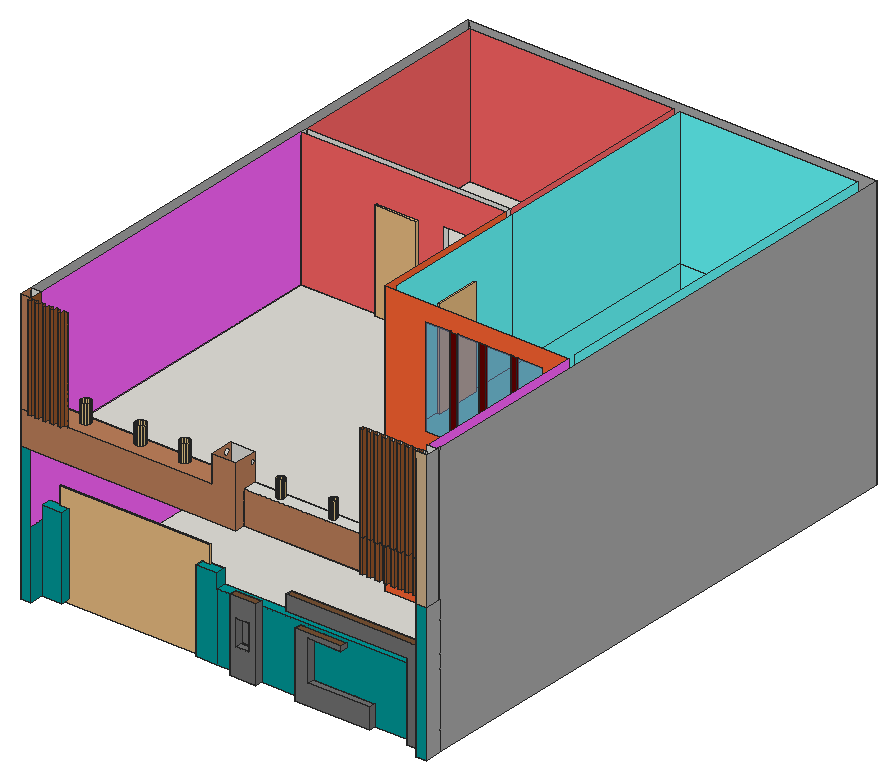
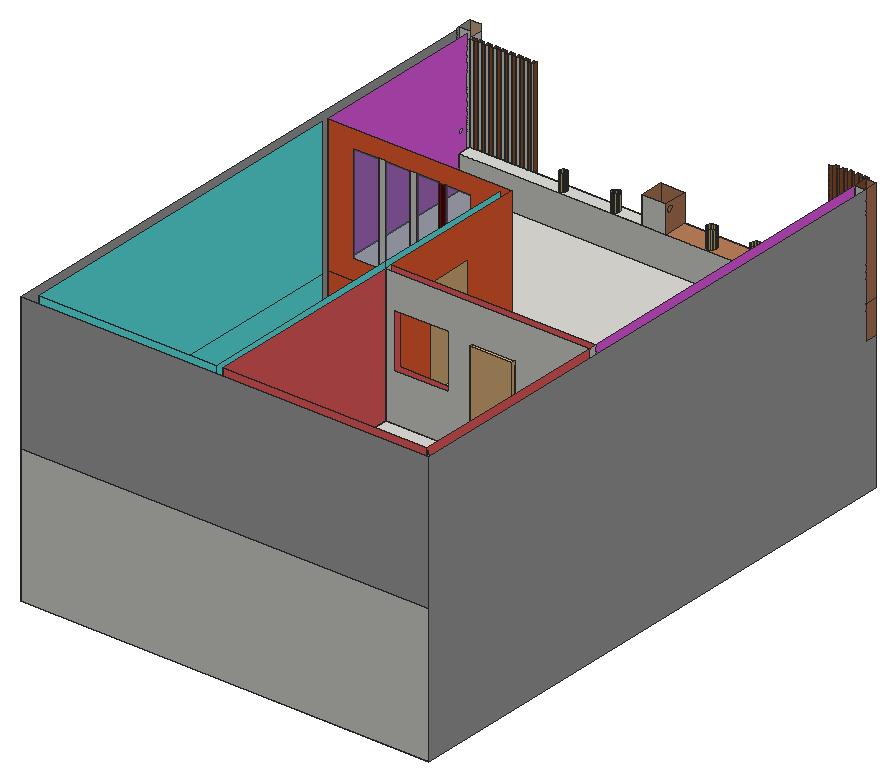
# SketchUp Ruby script. Lengths in inches.
U = 1.inch
M = Sketchup.active_model
def pt(a) = Geom::Point3d.new(a.map { |v| v * U })
def face(e, loops, mat)
  f = e.add_face(loops[0].map { |a| pt(a) })
  loops[1..].each { |l| e.add_face(l.map { |a| pt(a) }).erase! }
  f.material = f.back_material = mat if mat
  f
end
# faces: each face lists its corners as indices into pts; further lists are holes
def faces(e, pts, list, mat = nil) = list.each { |f| face(e, (f[0].is_a?(Array) ? f : [f]).map { |l| l.map { |i| pts[i] } }, mat) }
# xy, xz, yz: faces in a plane at the given z, y or x. An outline is a flat list of corners, or four numbers for a rectangle; further outlines are holes
def ring(l) = l.size == 4 ? [[l[0], l[1]], [l[2], l[1]], [l[2], l[3]], [l[0], l[3]]] : l.each_slice(2).to_a
def flat(e, list, mat, &to3) = list.each { |f| face(e, (f[0].is_a?(Array) ? f : [f]).map { |l| ring(l).map { |u, v| to3.(u, v) } }, mat) }
def xy(e, z, list, mat = nil) = flat(e, list, mat) { |x, y| [x, y, z] }
def xz(e, y, list, mat = nil) = flat(e, list, mat) { |x, z| [x, y, z] }
def yz(e, x, list, mat = nil) = flat(e, list, mat) { |y, z| [x, y, z] }
def lines(e, pts, list) = list.each { |a, b| e.add_line(pt(pts[a]), pt(pts[b])) }
# prism: a flat outline (further loops are holes) pulled along v
def prism(e, loops, v, mat = nil)
  f = face(e, loops, mat); d = Geom::Vector3d.new(v.map { |x| x * U })
  f.pushpull(f.normal.samedirection?(d) ? d.length : -d.length)
end
def box(e, o, s, mat = nil) = prism(e, [[o, [o[0] + s[0], o[1], o[2]], [o[0] + s[0], o[1] + s[1], o[2]], [o[0], o[1] + s[1], o[2]]]], [0, 0, s[2]], mat)
def at(x, y, z, deg = 0) = Geom::Transformation.translation(pt([x, y, z])) * Geom::Transformation.rotation(ORIGIN, Z_AXIS, deg.degrees)
def axes(o, x, y, z) = Geom::Transformation.new([*x, 0, *y, 0, *z, 0, *pt(o).to_a, 1])
def part(name) = M.definitions.add(name)
# library, detail: a bought-in or finely detailed component or shape, given as its bounding box
def library(name, o, s) = part(name).tap { |d| box(d.entities, o, s) }
def detail(e, o, s) = box(e.add_group.entities, o, s)
def put(e, d, t, mat = nil) = e.add_instance(d, t).tap { |i| i.material = mat if mat }
def group(e, t, mat = nil) = e.add_group.tap { |g| g.transformation = t; g.material = mat if mat }.entities
root = M.entities
M.materials.add("[0035_Tan]").color = [210, 180, 140]
M.materials.add("[Color A03]").color = [255, 101, 101]
M.materials.add("[Color A08]1").color = [102, 0, 0]
M.materials.add("[Color B04]").color = [255, 101, 50]
M.materials.add("[Color H03]").color = [101, 255, 255]
M.materials.add("[Color H07]").color = [0, 153, 153]
M.materials.add("[Color K03]").color = [255, 101, 255]
M.materials.add("[Color M03]").color = [170, 170, 170]
M.materials.add("[Color M05]").color = [114, 114, 114]
M.materials.add("[Color M09]").color = [0, 0, 0]
M.materials.add("[Marble Carrara Gold Floor Tile]").color = [225, 223, 217]
M.materials.add("[Sandstone]").color = [118, 81, 52]
M.materials.add("[Stone Brushed Khaki]").color = [226, 197, 133]
M.materials.add("[Translucent Glass Sky Reflection]").color = [126, 138, 183]
M.materials["[Translucent Glass Sky Reflection]"].alpha = 0.52
M.materials.add("[Wood Cherry Original]").color = [152, 86, 42]
M.materials.add("[Wood Veneer 02]").color = [190, 128, 91]
c1 = library("gate",[-28.22,15.88,-5.11],[182.45,4.03,139.23])
c2 = library("DOOR (1)\#1",[0,-8.5,0],[36,11.125,84])
c3 = library("DOOR (1)\#2",[0,-8.5,0],[36,11.125,84])
c4 = library("DOOR (1)",[0,-8.63,0],[36.49,11.68,86.95])
xy(root,0,[[351.25,24,360.25,39],[0.25,27,0.25,519,360.25,519,360.25,39,145.0625,39,145.0625,48,351.25,48,351.25,192.3125,188.875,192.3125,188.875,246.36,194.875,246.36,194.875,198.3125,351.25,198.3125,351.25,510,194.875,510,194.875,282.36,188.875,282.36,188.875,510,9.25,510,9.25,48,27.11,48,27.11,39,9.25,39,9.25,27],[9.25,324.96,75.75,330.96],[111.75,324.96,188.875,330.96]])
xy(root,0,[[9.25,48,351.25,48,351.25,192.3125,188.875,192.3125,188.875,246.36,194.875,246.36,194.875,282.36,188.875,282.36,188.875,324.96,111.75,324.96,111.75,330.96,75.75,330.96,75.75,324.96,9.25,324.96],[194.875,198.3125,351.25,510],[9.25,330.96,188.875,510]],"[Marble Carrara Gold Floor Tile]")
xy(root,0,[[180.02,33,203.03,39],[237.34,33,302.96,39],[335.59,33,351.25,39]],"[Sandstone]")
xy(root,17.83,[[248.65,33,302.96,39]],"[Color M05]")
xy(root,17.875,[[246.73,191.3125,252.73,192.3125],[272.86,191.3125,278.86,192.3125],[300.23,191.3125,306.23,192.3125]])
xy(root,24.41,[[185.3125,33,196.5,39]],"[Color M05]")
xy(root,41.89,[[133.81,324.96,181.81,330.96]])
xy(root,47.22,[[185.3125,33,196.5,39]],"[Color M05]")
xy(root,53.16,[[248.65,33,278.03,39]],"[Color M05]")
xy(root,57.34,[[237.34,33,278.03,39]],"[Sandstone]")
xy(root,60,[[163.53,39,351.25,48]],"[Color H07]")
xy(root,64.125,[[180.02,33,203.03,39]],"[Sandstone]")
xy(root,68.2,[[229.59,33,335.59,39]],"[Color M05]")
xy(root,72,[[9.25,39,27.11,48],[145.0625,39,163.53,48]],"[Color H07]")
xy(root,81.18,[[229.59,33,351.25,39]],"[Sandstone]")
xy(root,84,[[188.875,246.36,194.875,282.36],[75.75,324.96,111.75,330.96]])
xy(root,89.89,[[133.81,324.96,181.81,330.96]])
xy(root,104.8125,[[246.73,191.3125,252.73,192.3125],[272.86,191.3125,278.86,192.3125],[300.23,191.3125,306.23,192.3125]],"[Color A08]1")
xy(root,120,[[351.25,24,360.25,36],[351.25,36,360.25,39],[9.25,39,351.25,48],[188.875,282.36,188.875,330.375,194.875,324.375,194.875,282.36],[9.25,324.96,75.75,330.96],
  [111.75,324.96,188.875,324.96,188.875,330.375,188.29,330.96,111.75,330.96],[188.875,330.375,188.875,330.96,188.29,330.96]])
xy(root,120,[[75.75,324.96,111.75,330.96]],"[Color A03]")
xy(root,120,[[188.875,246.36,194.875,282.36]],"[Color B04]")
xy(root,120,[[9.25,48,351.25,48,351.25,192.3125,188.875,192.3125,188.875,324.96,9.25,324.96],[9.25,330.96,188.875,510]],"[Marble Carrara Gold Floor Tile]")
xy(root,120,[[294.16,33,296.82,36],[300.5,33,304.19,36],[307.88,33,311.57,36],[315.25,33,318.44,36],[321.63,33,324.82,36],
  [328,33,331.19,36],[334.38,33,337.57,36],[340.75,33,343.94,36],[347.13,33,351.25,36]],"[Wood Cherry Original]")
xy(root,120,[[9.25,27,190.02,39],[190.02,36,351.25,39]],"[Wood Veneer 02]")
xy(root,137.875,[[246.73,191.3125,252.73,192.3125],[272.86,191.3125,278.86,192.3125],[300.23,191.3125,306.23,192.3125]])
xy(root,149.4375,[[0.25,27,9.25,39],[294.16,33,296.82,36],[300.5,33,303.66,36],[307.88,33,310.41,36],[315.25,33,317.16,36],
  [321.63,33,323.91,36],[328,33,330.66,36],[334.38,33,337.41,36],[337.41,33,337.57,36],[340.75,33,340.79,36],
  [340.79,33,343.94,36],[343.94,33,344.16,36],[347.13,33,351.25,36],[[190.02,36,351.25,48],[217.02,39.6875,216.19,39.77,215.42,40.0625,214.74,40.55,214.21,41.19,213.87,41.95,213.74,42.77,213.82,43.6,214.11,44.38,214.6,45.05,215.24,45.58,216,45.92,216.82,46.06,217.65,45.98,218.43,45.68,219.1,45.2,219.63,44.55,219.97,43.79,220.11,42.97,220.03,42.14,219.73,41.37,219.25,40.69,218.6,40.16,217.84,39.82],[263.46,39.6875,262.63,39.77,261.85,40.0625,261.18,40.55,260.65,41.19,260.31,41.95,260.17,42.77,260.26,43.6,260.55,44.38,261.04,45.05,261.68,45.58,262.4375,45.92,263.26,46.06,264.09,45.98,264.87,45.68,265.54,45.2,266.07,44.55,266.41,43.79,266.55,42.97,266.46,42.14,266.17,41.37,265.68,40.69,265.04,40.16,264.28,39.82]],[94.51,37.09,93.375,37.24,92.32,37.68,91.41,38.375,90.72,39.28,90.28,40.34,90.13,41.47,90.28,42.6,90.72,43.66,91.41,44.56,92.32,45.26,93.375,45.7,94.51,45.85,95.64,45.7,96.7,45.26,97.6,44.56,98.3,43.66,98.74,42.6,98.89,41.47,98.74,40.34,98.3,39.28,97.6,38.375,96.7,37.68,95.64,37.24],
  [133.45,37.09,132.3125,37.24,131.26,37.68,130.35,38.375,129.66,39.28,129.22,40.34,129.07,41.47,129.22,42.6,129.66,43.66,130.35,44.56,131.26,45.26,132.3125,45.7,133.45,45.85,134.58,45.7,135.64,45.26,136.54,44.56,137.24,43.66,137.67,42.6,137.82,41.47,137.67,40.34,137.24,39.28,136.54,38.375,135.64,37.68,134.58,37.24],[217.02,39.6875,216.19,39.77,215.42,40.0625,214.74,40.55,214.21,41.19,213.87,41.95,213.74,42.77,213.82,43.6,214.11,44.38,214.6,45.05,215.24,45.58,216,45.92,216.82,46.06,217.65,45.98,218.43,45.68,219.1,45.2,219.63,44.55,219.97,43.79,220.11,42.97,220.03,42.14,219.73,41.37,219.25,40.69,218.6,40.16,217.84,39.82],[263.46,39.6875,262.63,39.77,261.85,40.0625,261.18,40.55,260.65,41.19,260.31,41.95,260.17,42.77,260.26,43.6,260.55,44.38,261.04,45.05,261.68,45.58,262.4375,45.92,263.26,46.06,264.09,45.98,264.87,45.68,265.54,45.2,266.07,44.55,266.41,43.79,266.55,42.97,266.46,42.14,266.17,41.37,265.68,40.69,265.04,40.16,264.28,39.82]])
xy(root,149.4375,[[9.25,24,12.5,27],[15.75,24,19,27],[22.25,24,25.5,27],[28.75,24,32,27],[35.25,24,38.5,27],
  [296.82,33,296.91,36],[300.29,33,300.5,36],[303.66,33,304.19,36],[307.04,33,307.88,36],[310.41,33,311.57,36],
  [313.79,33,315.25,36],[317.16,33,318.44,36],[320.54,33,321.63,36],[323.91,33,324.82,36],[327.29,33,328,36],
  [330.66,33,331.19,36],[334.04,33,334.38,36]],"[Wood Cherry Original]")
xy(root,149.4375,[[[9.25,27,169.02,48],[133.45,37.09,132.3125,37.24,131.26,37.68,130.35,38.375,129.66,39.28,129.22,40.34,129.07,41.47,129.22,42.6,129.66,43.66,130.35,44.56,131.26,45.26,132.3125,45.7,133.45,45.85,134.58,45.7,135.64,45.26,136.54,44.56,137.24,43.66,137.67,42.6,137.82,41.47,137.67,40.34,137.24,39.28,136.54,38.375,135.64,37.68,134.58,37.24],[94.51,37.09,93.375,37.24,92.32,37.68,91.41,38.375,90.72,39.28,90.28,40.34,90.13,41.47,90.28,42.6,90.72,43.66,91.41,44.56,92.32,45.26,93.375,45.7,94.51,45.85,95.64,45.7,96.7,45.26,97.6,44.56,98.3,43.66,98.74,42.6,98.89,41.47,98.74,40.34,98.3,39.28,97.6,38.375,96.7,37.68,95.64,37.24],[46.45,37.09,45.3125,37.24,44.26,37.68,43.35,38.375,42.66,39.28,42.22,40.34,42.07,41.47,42.22,42.6,42.66,43.66,43.35,44.56,44.26,45.26,45.3125,45.7,46.45,45.85,47.58,45.7,48.64,45.26,49.54,44.56,50.24,43.66,50.67,42.6,50.82,41.47,50.67,40.34,50.24,39.28,49.54,38.375,48.64,37.68,47.58,37.24]]],"[Wood Veneer 02]")
xz(root,24,[[351.25,120,360.25,240.8125]],"[0035_Tan]")
xz(root,24,[[351.25,0,360.25,120]],"[Color H07]")
xz(root,24,[[9.25,149.4375,12.5,240],[15.75,149.4375,19,240],[22.25,149.4375,25.5,240],[28.75,149.4375,32,240],[35.25,149.4375,38.5,240]],"[Wood Cherry Original]")
xz(root,27,[[9.25,149.4375,12.5,240]])
xz(root,27,[[0.25,0,9.25,120]],"[Color H07]")
xz(root,27,[[12.5,149.4375,15.75,240],[19,149.4375,22.25,240],[25.5,149.4375,28.75,240],[32,149.4375,35.25,240],[38.5,149.4375,41.75,240],
  [41.75,149.4375,42.3125,240]],"[Wood Cherry Original]")
xz(root,27,[[0.25,120,190.02,120,190.02,173.4375,169.02,173.4375,169.02,149.4375,0.25,149.4375],[0.25,149.4375,9.25,240]],"[Wood Veneer 02]")
xz(root,33,[[[180.02,0,203.03,64.125],[185.3125,24.41,196.5,47.22]],[335.59,0,351.25,0,351.25,81.18,229.59,81.18,229.59,68.2,335.59,68.2],[237.34,0,302.96,0,302.96,17.83,248.65,17.83,248.65,53.16,278.03,53.16,278.03,57.34,237.34,57.34]],"[Color M05]")
xz(root,33,[[294.16,120,296.82,149.4375],[300.5,120,304.19,149.4375],[307.88,120,311.57,149.4375],[315.25,120,318.44,149.4375],[321.63,120,324.82,149.4375],
  [328,120,331.19,149.4375],[334.38,120,337.57,149.4375],[340.75,120,343.94,149.4375],[347.13,120,351.25,149.4375],[294.16,149.4375,296.91,234.8125],
  [300.29,149.4375,303.66,234.8125],[307.04,149.4375,310.41,234.8125],[313.79,149.4375,317.16,234.8125],[320.54,149.4375,323.91,234.8125],[327.29,149.4375,330.66,234.8125],
  [334.04,149.4375,337.41,234.8125],[340.79,149.4375,344.16,234.8125],[347.13,149.4375,351.25,234.8125]],"[Wood Cherry Original]")
xz(root,36,[[294.16,120,296.82,149.4375],[300.5,120,304.19,149.4375],[307.88,120,311.57,149.4375],[315.25,120,318.44,149.4375],[321.63,120,324.82,149.4375],
  [328,120,331.19,149.4375],[334.38,120,337.57,149.4375],[340.75,120,343.94,149.4375],[347.13,120,351.25,149.4375],[351.25,120,360.25,240.8125],
  [294.16,149.4375,296.91,234.8125],[300.29,149.4375,303.66,234.8125],[307.04,149.4375,310.41,234.8125],[313.79,149.4375,317.16,234.8125],[320.54,149.4375,323.91,234.8125],
  [327.29,149.4375,330.66,234.8125],[334.04,149.4375,337.41,234.8125],[340.79,149.4375,344.16,234.8125],[347.13,149.4375,351.25,234.8125]])
xz(root,36,[[296.82,120,300.5,149.4375],[304.19,120,307.88,149.4375],[311.57,120,315.25,149.4375],[318.44,120,321.63,149.4375],[324.82,120,328,149.4375],
  [331.19,120,334.38,149.4375],[337.57,120,340.75,149.4375],[343.94,120,347.13,149.4375],[296.91,149.4375,300.29,234.8125],[303.66,149.4375,307.04,234.8125],
  [310.41,149.4375,313.79,234.8125],[317.16,149.4375,320.54,234.8125],[323.91,149.4375,327.29,234.8125],[330.66,149.4375,334.04,234.8125],[337.41,149.4375,340.79,234.8125],
  [344.16,149.4375,347.13,234.8125]],"[Wood Cherry Original]")
xz(root,36,[[190.02,120,294.16,149.4375]],"[Wood Veneer 02]")
xz(root,39,[[[180.02,0,203.03,60],[185.3125,24.41,196.5,47.22]],[237.34,0,237.34,57.34,278.03,57.34,278.03,53.16,248.65,53.16,248.65,17.83,302.96,17.83,302.96,0],[335.59,0,351.25,60],[351.25,0,360.25,120],[180.02,60,203.03,64.125],
  [335.59,60,335.59,68.2,229.59,68.2,229.59,81.18,351.25,81.18,351.25,60],[0.25,149.4375,9.25,240]])
xz(root,39,[[9.25,0,27.11,72],[145.0625,0,163.53,72],[163.53,0,180.02,60],[203.03,0,237.34,0,237.34,57.34,278.03,57.34,278.03,53.16,248.65,53.16,248.65,17.83,302.96,17.83,302.96,0,335.59,0,335.59,60,203.03,60]],"[Color H07]")
xz(root,39,[[185.3125,24.41,196.5,47.22]],"[Color M05]")
xz(root,48,[[9.25,0,27.11,72],[145.0625,0,145.0625,72,163.53,72,163.53,60,351.25,60,351.25,0],[9.25,120,351.25,149.4375],[169.02,149.4375,190.02,173.4375]])
xz(root,191.3125,[[246.73,17.875,252.73,104.8125],[272.86,17.875,278.86,104.8125],[300.23,17.875,306.23,104.8125],[246.73,137.875,252.73,224.8125],[272.86,137.875,278.86,224.8125],
  [300.23,137.875,306.23,224.8125]],"[Color A08]1")
xz(root,192.3125,[[272.86,17.875,278.86,104.8125],[300.23,17.875,306.23,104.8125],[272.86,137.875,278.86,224.8125],[300.23,137.875,306.23,224.8125]])
xz(root,192.3125,[[[188.875,0,351.25,120],[224.8,17.875,328.11,104.8125]],[[188.875,120,351.25,240],[224.8,137.875,328.11,224.8125]]],"[Color B04]")
xz(root,192.3125,[[224.8,17.875,246.73,104.8125],[252.73,17.875,272.86,104.8125],[278.86,17.875,300.23,104.8125],[306.23,17.875,328.11,104.8125],[224.8,137.875,246.73,224.8125],
  [252.73,137.875,272.86,224.8125],[278.86,137.875,300.23,224.8125],[306.23,137.875,328.11,224.8125]],"[Translucent Glass Sky Reflection]")
xz(root,246.36,[[188.875,0,194.875,84],[188.875,120,194.875,204]])
xz(root,282.36,[[188.875,0,194.875,84],[188.875,120,194.875,204]])
xz(root,324.96,[[[9.25,0,75.75,0,75.75,84,111.75,84,111.75,0,188.875,0,188.875,120,9.25,120],[133.81,41.89,181.81,89.89]],[[9.25,120,75.75,120,75.75,204,111.75,204,111.75,120,188.875,120,188.875,240,9.25,240],[133.81,161.89,181.81,209.89]]],"[Color A03]")
xz(root,330.96,[[[9.25,0,9.25,120,188.875,120,188.875,0,111.75,0,111.75,84,75.75,84,75.75,0],[133.81,41.89,181.81,89.89]],[[9.25,120,9.25,240,188.875,240,188.875,120,111.75,120,111.75,204,75.75,204,75.75,120],[133.81,161.89,181.81,209.89]]])
xz(root,510,[[9.25,0,188.875,120],[9.25,120,188.875,240]],"[Color A03]")
xz(root,510,[[194.875,0,351.25,120],[194.875,120,351.25,240]],"[Color H03]")
xz(root,519,[[0.25,0,360.25,120]])
xz(root,519,[[0.25,120,360.25,240]],"[Color M03]")
yz(root,0.25,[[27,0,27,120,39,120,39,240,519,240,519,0]],"[Color M03]")
yz(root,0.25,[[27,120,39,149.4375],[27,149.4375,39,240]],"[Wood Veneer 02]")
yz(root,9.25,[[324.96,0,330.96,120],[324.96,120,330.96,240]])
yz(root,9.25,[[330.96,0,510,120],[330.96,120,510,240]],"[Color A03]")
yz(root,9.25,[[27,0,39,60]],"[Color H07]")
yz(root,9.25,[[48,0,324.96,0,324.96,120,27,120,27,60,39,60,39,72,48,72],[48,120,324.96,120,324.96,240,39,240,39,149.4375,48,149.4375]],"[Color K03]")
yz(root,9.25,[[24,149.4375,27,240],[27,149.4375,39,240]],"[Wood Cherry Original]")
yz(root,12.5,[[24,149.4375,27,240]],"[Wood Cherry Original]")
yz(root,15.75,[[24,149.4375,27,240]],"[Wood Cherry Original]")
yz(root,19,[[24,149.4375,27,240]],"[Wood Cherry Original]")
yz(root,22.25,[[24,149.4375,27,240]],"[Wood Cherry Original]")
yz(root,25.5,[[24,149.4375,27,240]],"[Wood Cherry Original]")
yz(root,27.11,[[39,0,48,72]],"[Color H07]")
yz(root,28.75,[[24,149.4375,27,240]],"[Wood Cherry Original]")
yz(root,32,[[24,149.4375,27,240]],"[Wood Cherry Original]")
yz(root,35.25,[[24,149.4375,27,240]],"[Wood Cherry Original]")
yz(root,38.5,[[24,149.4375,27,240]],"[Wood Cherry Original]")
yz(root,75.75,[[324.96,0,330.96,84],[324.96,120,330.96,204]])
yz(root,111.75,[[324.96,0,330.96,84],[324.96,120,330.96,204]])
yz(root,133.81,[[324.96,41.89,330.96,89.89]])
yz(root,145.0625,[[39,0,48,60],[39,60,48,72]],"[Color H07]")
yz(root,163.53,[[39,60,48,72]],"[Color H07]")
yz(root,169.02,[[[27,149.4375,48,173.4375],[43.19,164.77,43.99,164.88,44.73,165.18,45.36,165.67,45.85,166.3,46.15,167.04,46.26,167.84,46.15,168.63,45.85,169.37,45.36,170,44.73,170.49,43.99,170.79,43.19,170.9,42.4,170.79,41.66,170.49,41.03,170,40.54,169.37,40.24,168.63,40.13,167.84,40.24,167.04,40.54,166.3,41.03,165.67,41.66,165.18,42.4,164.88]]],"[Wood Veneer 02]")
yz(root,180.02,[[33,0,39,64.125]],"[Color M05]")
yz(root,181.81,[[324.96,41.89,330.96,89.89]])
yz(root,185.3125,[[33,24.41,39,47.22]],"[Color M05]")
yz(root,188.875,[[324.96,0,330.96,120],[324.96,120,330.96,240]])
yz(root,188.875,[[330.96,0,510,120],[330.96,120,510,240]],"[Color A03]")
yz(root,188.875,[[192.3125,0,192.3125,120,324.96,120,324.96,0,282.36,0,282.36,84,246.36,84,246.36,0],[192.3125,120,192.3125,240,324.96,240,324.96,120,282.36,120,282.36,204,246.36,204,246.36,120]],"[Color B04]")
yz(root,190.02,[[36,120,39,149.4375]])
yz(root,190.02,[[[27,120,36,120,36,149.4375,48,149.4375,48,173.4375,27,173.4375],[45.4,163.94,44.83,164.02,44.3,164.24,43.85,164.58,43.5,165.04,43.28,165.5625,43.21,166.13,43.28,166.7,43.5,167.22,43.85,167.68,44.3,168.02,44.83,168.24,45.4,168.32,45.96,168.24,46.49,168.02,46.94,167.68,47.29,167.22,47.51,166.7,47.58,166.13,47.51,165.5625,47.29,165.04,46.94,164.58,46.49,164.24,45.96,164.02]]],"[Wood Veneer 02]")
yz(root,194.875,[[198.3125,0,246.36,0,246.36,84,282.36,84,282.36,0,510,0,510,120,198.3125,120],[198.3125,120,246.36,120,246.36,204,282.36,204,282.36,120,324.375,120,324.375,240,198.3125,240],[324.375,120,510,240]],"[Color H03]")
yz(root,196.5,[[33,24.41,39,47.22]],"[Color M05]")
yz(root,203.03,[[33,0,39,64.125]],"[Color M05]")
yz(root,229.59,[[33,68.2,39,81.18]],"[Color M05]")
yz(root,237.34,[[33,0,39,57.34]],"[Color M05]")
yz(root,246.73,[[191.3125,17.875,192.3125,104.8125],[191.3125,137.875,192.3125,224.8125]],"[Color A08]1")
yz(root,248.65,[[33,17.83,39,53.16]],"[Color M05]")
yz(root,252.73,[[191.3125,17.875,192.3125,104.8125],[191.3125,137.875,192.3125,224.8125]],"[Color A08]1")
yz(root,272.86,[[191.3125,17.875,192.3125,104.8125],[191.3125,137.875,192.3125,224.8125]],"[Color A08]1")
yz(root,278.03,[[33,53.16,39,57.34]],"[Color M05]")
yz(root,278.86,[[191.3125,17.875,192.3125,104.8125],[191.3125,137.875,192.3125,224.8125]],"[Color A08]1")
yz(root,294.16,[[33,120,36,149.4375],[33,149.4375,36,234.8125]],"[Wood Cherry Original]")
yz(root,296.82,[[33,120,36,149.4375]],"[Wood Cherry Original]")
yz(root,296.91,[[33,149.4375,36,234.8125]],"[Wood Cherry Original]")
yz(root,300.23,[[191.3125,17.875,192.3125,104.8125],[191.3125,137.875,192.3125,224.8125]],"[Color M09]")
yz(root,300.29,[[33,149.4375,36,234.8125]],"[Wood Cherry Original]")
yz(root,300.5,[[33,120,36,149.4375]],"[Wood Cherry Original]")
yz(root,302.96,[[33,0,39,17.83]],"[Color M05]")
yz(root,303.66,[[33,149.4375,36,234.8125]],"[Wood Cherry Original]")
yz(root,304.19,[[33,120,36,149.4375]],"[Wood Cherry Original]")
yz(root,306.23,[[191.3125,17.875,192.3125,104.8125],[191.3125,137.875,192.3125,224.8125]],"[Color A08]1")
yz(root,307.04,[[33,149.4375,36,234.8125]],"[Wood Cherry Original]")
yz(root,307.88,[[33,120,36,149.4375]],"[Wood Cherry Original]")
yz(root,310.41,[[33,149.4375,36,234.8125]],"[Wood Cherry Original]")
yz(root,311.57,[[33,120,36,149.4375]],"[Wood Cherry Original]")
yz(root,313.79,[[33,149.4375,36,234.8125]],"[Wood Cherry Original]")
yz(root,315.25,[[33,120,36,149.4375]],"[Wood Cherry Original]")
yz(root,317.16,[[33,149.4375,36,234.8125]],"[Wood Cherry Original]")
yz(root,318.44,[[33,120,36,149.4375]],"[Wood Cherry Original]")
yz(root,320.54,[[33,149.4375,36,234.8125]],"[Wood Cherry Original]")
yz(root,321.63,[[33,120,36,149.4375]],"[Wood Cherry Original]")
yz(root,323.91,[[33,149.4375,36,234.8125]],"[Wood Cherry Original]")
yz(root,324.82,[[33,120,36,149.4375]],"[Wood Cherry Original]")
yz(root,327.29,[[33,149.4375,36,234.8125]],"[Wood Cherry Original]")
yz(root,328,[[33,120,36,149.4375]],"[Wood Cherry Original]")
yz(root,330.66,[[33,149.4375,36,234.8125]],"[Wood Cherry Original]")
yz(root,331.19,[[33,120,36,149.4375]],"[Wood Cherry Original]")
yz(root,334.04,[[33,149.4375,36,234.8125]],"[Wood Cherry Original]")
yz(root,334.38,[[33,120,36,149.4375]],"[Wood Cherry Original]")
yz(root,335.59,[[33,0,39,68.2]],"[Color M05]")
yz(root,337.41,[[33,149.4375,36,234.8125]],"[Wood Cherry Original]")
yz(root,337.57,[[33,120,36,149.4375]],"[Wood Cherry Original]")
yz(root,340.75,[[33,120,36,149.4375]],"[Wood Cherry Original]")
yz(root,340.79,[[33,149.4375,36,234.8125]],"[Wood Cherry Original]")
yz(root,343.94,[[33,120,36,149.4375]],"[Wood Cherry Original]")
yz(root,344.16,[[33,149.4375,36,234.8125]],"[Wood Cherry Original]")
yz(root,347.13,[[33,120,36,149.4375],[33,149.4375,36,234.8125]],"[Wood Cherry Original]")
yz(root,351.25,[[33,0,39,81.18],[24,120,33,234.8125],[33,120,36,149.4375],[36,120,48,149.4375],[33,149.4375,36,234.8125],
  [36,149.4375,39,234.8125]])
yz(root,351.25,[[198.3125,0,510,120],[198.3125,120,510,240]],"[Color H03]")
yz(root,351.25,[[24,0,33,60],[24,60,24,120,39,120,39,81.18,33,81.18,33,60]],"[Color H07]")
yz(root,351.25,[[48,0,48,60,39,60,39,120,192.3125,120,192.3125,0],[[48,120,48,149.4375,39,149.4375,39,240,192.3125,240,192.3125,120],[45.4,163.94,45.96,164.02,46.49,164.24,46.94,164.58,47.29,165.04,47.51,165.5625,47.58,166.13,47.51,166.7,47.29,167.22,46.94,167.68,46.49,168.02,45.96,168.24,45.4,168.32,44.83,168.24,44.3,168.02,43.85,167.68,43.5,167.22,43.28,166.7,43.21,166.13,43.28,165.5625,43.5,165.04,43.85,164.58,44.3,164.24,44.83,164.02]]],"[Color K03]")
yz(root,360.25,[[24,0,39,120],[39,0,519,240],[24,120,36,240.8125],[36,120,39,240.9375]],"[Color M03]")
p = [[0.25,519,120],[0.25,519,240],[9.25,510,240],[9.25,510,120],[45.3125,37.24,149.4375],[46.45,37.09,149.4375],
  [46.45,37.09,165.67],[45.3125,37.24,165.67],[47.58,37.24,149.4375],[47.58,37.24,165.67],[93.375,37.24,149.4375],[94.51,37.09,149.4375],
  [94.51,37.09,165.0625],[93.375,37.24,165.0625],[95.64,37.24,149.4375],[95.64,37.24,165.0625],[132.3125,37.24,149.4375],[133.45,37.09,149.4375],
  [133.45,37.09,164.88],[132.3125,37.24,164.88],[134.58,37.24,149.4375],[134.58,37.24,164.88],[44.26,37.68,149.4375],[44.26,37.68,165.67],
  [48.64,37.68,149.4375],[48.64,37.68,165.67],[92.32,37.68,149.4375],[92.32,37.68,165.0625],[96.7,37.68,149.4375],[96.7,37.68,165.0625],
  [131.26,37.68,149.4375],[131.26,37.68,164.88],[135.64,37.68,149.4375],[135.64,37.68,164.88],[43.35,38.375,149.4375],[43.35,38.375,165.67],
  [49.54,38.375,149.4375],[49.54,38.375,165.67],[91.41,38.375,149.4375],[91.41,38.375,165.0625],[97.6,38.375,149.4375],[97.6,38.375,165.0625],
  [130.35,38.375,149.4375],[130.35,38.375,164.88],[136.54,38.375,149.4375],[136.54,38.375,164.88],[42.66,39.28,149.4375],[42.66,39.28,165.67],
  [50.24,39.28,149.4375],[50.24,39.28,165.67],[90.72,39.28,149.4375],[90.72,39.28,165.0625],[98.3,39.28,149.4375],[98.3,39.28,165.0625],
  [129.66,39.28,149.4375],[129.66,39.28,164.88],[137.24,39.28,149.4375],[137.24,39.28,164.88],[42.22,40.34,149.4375],[42.22,40.34,165.67],
  [50.67,40.34,149.4375],[50.67,40.34,165.67],[90.28,40.34,149.4375],[90.28,40.34,165.0625],[98.74,40.34,149.4375],[98.74,40.34,165.0625],
  [129.22,40.34,149.4375],[129.22,40.34,164.88],[137.67,40.34,149.4375],[137.67,40.34,164.88],[216.19,39.77,149.4375],[217.02,39.6875,149.4375],
  [217.02,39.6875,164.24],[216.19,39.77,164.24],[217.84,39.82,149.4375],[217.84,39.82,164.24],[262.63,39.77,149.4375],[263.46,39.6875,149.4375],
  [263.46,39.6875,163.8125],[262.63,39.77,163.8125],[264.28,39.82,149.4375],[264.28,39.82,163.8125],[215.42,40.0625,149.4375],[215.42,40.0625,164.24],
  [218.6,40.16,149.4375],[218.6,40.16,164.24],[261.85,40.0625,149.4375],[261.85,40.0625,163.8125],[265.04,40.16,149.4375],[265.04,40.16,163.8125],
  [214.74,40.55,149.4375],[214.74,40.55,164.24],[261.18,40.55,149.4375],[261.18,40.55,163.8125],[219.25,40.69,149.4375],[219.25,40.69,164.24],
  [265.68,40.69,149.4375],[265.68,40.69,163.8125],[42.07,41.47,149.4375],[42.13,41.03,165.67],[42.07,41.47,165.67],[50.82,41.47,149.4375],
  [50.82,41.47,165.67],[50.77,41.03,165.67],[90.13,41.47,149.4375],[90.13,41.47,165.0625],[98.89,41.47,149.4375],[98.89,41.47,165.0625],
  [129.07,41.47,149.4375],[129.07,41.47,164.88],[137.82,41.47,149.4375],[137.82,41.47,164.88],[214.21,41.19,149.4375],[214.21,41.19,164.24],
  [260.65,41.19,149.4375],[260.65,41.19,163.8125],[219.73,41.37,149.4375],[219.73,41.37,164.24],[266.17,41.37,149.4375],[266.17,41.37,163.8125],
  [213.87,41.95,149.4375],[213.87,41.95,164.24],[260.31,41.95,149.4375],[260.31,41.95,163.8125],[220.03,42.14,149.4375],[220.03,42.14,164.24],
  [266.46,42.14,149.4375],[266.46,42.14,163.8125],[42.22,42.6,149.4375],[42.22,42.6,165.67],[50.67,42.6,149.4375],[50.67,42.6,165.67],
  [90.28,42.6,149.4375],[90.28,42.6,165.0625],[98.74,42.6,149.4375],[98.74,42.6,165.0625],[129.22,42.6,149.4375],[129.19,42.4,164.88],
  [129.22,42.6,164.88],[137.67,42.6,149.4375],[137.67,42.6,164.88],[137.7,42.4,164.88],[213.74,42.77,149.4375],[213.74,42.77,164.24],
  [260.17,42.77,149.4375],[260.17,42.77,163.8125],[220.11,42.97,149.4375],[220.11,42.97,164.24],[266.55,42.97,149.4375],[266.55,42.97,163.8125],
  [42.66,43.66,149.4375],[42.66,43.66,165.67],[50.24,43.66,149.4375],[50.24,43.66,165.67],[90.72,43.66,149.4375],[90.72,43.66,165.0625],
  [98.3,43.66,149.4375],[98.3,43.66,165.0625],[129.66,43.66,149.4375],[129.66,43.66,164.88],[137.24,43.66,149.4375],[137.24,43.66,164.88],
  [213.82,43.6,149.4375],[213.82,43.6,164.24],[260.26,43.6,149.4375],[260.26,43.6,163.8125],[219.97,43.79,149.4375],[219.97,43.79,164.24],
  [266.41,43.79,149.4375],[266.41,43.79,163.8125],[214.11,44.38,149.4375],[214.08,44.3,164.24],[214.11,44.38,164.24],[260.55,44.38,149.4375],
  [260.55,44.38,163.8125],[43.35,44.56,149.4375],[43.35,44.56,165.67],[49.54,44.56,149.4375],[49.54,44.56,165.67],[91.41,44.56,149.4375],
  [91.41,44.56,165.0625],[97.6,44.56,149.4375],[97.6,44.56,165.0625],[130.35,44.56,149.4375],[129.91,43.99,164.88],[130.35,44.56,164.88],
  [136.54,44.56,149.4375],[136.54,44.56,164.88],[136.99,43.99,164.88],[219.63,44.55,149.4375],[219.63,44.55,164.24],[219.74,44.3,164.24],
  [266.07,44.55,149.4375],[266.07,44.55,163.8125],[214.6,45.05,149.4375],[214.6,45.05,164.24],[261.04,45.05,149.4375],[261.04,45.05,163.8125],
  [44.26,45.26,149.4375],[44.26,45.26,165.67],[48.64,45.26,149.4375],[48.64,45.26,165.67],[92.32,45.26,149.4375],[92.32,45.26,165.0625],
  [96.7,45.26,149.4375],[96.7,45.26,165.0625],[131.26,45.26,149.4375],[131.26,45.26,164.88],[135.64,45.26,149.4375],[135.64,45.26,164.88],
  [219.1,45.2,149.4375],[219.1,45.2,164.24],[265.54,45.2,149.4375],[265.54,45.2,163.8125],[215.24,45.58,149.4375],[215.24,45.58,164.24],
  [261.68,45.58,149.4375],[261.68,45.58,163.8125],[218.43,45.68,149.4375],[218.43,45.68,164.24],[264.87,45.68,149.4375],[264.87,45.68,163.8125],
  [45.3125,45.7,149.4375],[44.5,45.36,165.67],[45.3125,45.7,165.67],[47.58,45.7,149.4375],[47.58,45.7,165.67],[48.39,45.36,165.67],
  [93.375,45.7,149.4375],[93.375,45.7,165.0625],[95.64,45.7,149.4375],[95.64,45.7,165.0625],[132.3125,45.7,149.4375],[132.3125,45.7,164.88],
  [134.58,45.7,149.4375],[134.58,45.7,164.88],[216,45.92,149.4375],[216,45.92,164.24],[262.4375,45.92,149.4375],[262.4375,45.92,163.8125],
  [46.45,45.85,149.4375],[46.45,45.85,165.67],[94.51,45.85,149.4375],[94.51,45.85,165.0625],[133.45,45.85,149.4375],[133.45,45.85,164.88],
  [217.65,45.98,149.4375],[217.65,45.98,164.24],[264.09,45.98,149.4375],[264.09,45.98,163.8125],[216.82,46.06,149.4375],[216.82,46.06,164.24],
  [263.26,46.06,149.4375],[263.26,46.06,163.8125],[157.81,324.96,89.89],[157.81,324.96,65.89],[133.81,324.96,65.89],[157.81,324.96,41.89],
  [181.81,324.96,65.89]]
faces(root,p,[[0,1,2,3]])
faces(root,p,[[4,5,6,7],[5,8,9,6],[10,11,12,13],[11,14,15,12],[16,17,18,19],[17,20,21,18],[22,4,7,23],[8,24,25,9],
  [26,10,13,27],[14,28,29,15],[30,16,19,31],[20,32,33,21],[34,22,23,35],[24,36,37,25],[38,26,27,39],[28,40,41,29],
  [42,30,31,43],[32,44,45,33],[46,34,35,47],[36,48,49,37],[50,38,39,51],[40,52,53,41],[54,42,43,55],[44,56,57,45],
  [58,46,47,59],[48,60,61,49],[62,50,51,63],[52,64,65,53],[66,54,55,67],[56,68,69,57],[70,71,72,73],[71,74,75,72],
  [76,77,78,79],[77,80,81,78],[82,70,73,83],[74,84,85,75],[86,76,79,87],[80,88,89,81],[90,82,83,91],[92,86,87,93],
  [84,94,95,85],[88,96,97,89],[98,58,59,99,100],[60,101,102,103,61],[104,62,63,105],[64,106,107,65],[108,66,67,109],[68,110,111,69],
  [112,90,91,113],[114,92,93,115],[94,116,117,95],[96,118,119,97],[120,112,113,121],[122,114,115,123],[116,124,125,117],[118,126,127,119],
  [128,98,100,129],[101,130,131,102],[132,104,105,133],[106,134,135,107],[136,108,109,137,138],[110,139,140,141,111],[142,120,121,143],[144,122,123,145],
  [124,146,147,125],[126,148,149,127],[150,128,129,151],[130,152,153,131],[154,132,133,155],[134,156,157,135],[158,136,138,159],[139,160,161,140],
  [162,142,143,163],[164,144,145,165],[146,166,167,147],[148,168,169,149],[170,162,163,171,172],[173,164,165,174],[175,150,151,176],[152,177,178,153],
  [179,154,155,180],[156,181,182,157],[183,158,159,184,185],[160,186,187,188,161],[166,189,190,191,167],[168,192,193,169],[194,170,172,195],[196,173,174,197],
  [198,175,176,199],[177,200,201,178],[202,179,180,203],[181,204,205,182],[206,183,185,207],[186,208,209,187],[189,210,211,190],[192,212,213,193],
  [214,194,195,215],[216,196,197,217],[210,218,219,211],[212,220,221,213],[222,198,199,223,224],[200,225,226,227,201],[228,202,203,229],[204,230,231,205],
  [232,206,207,233],[208,234,235,209],[236,214,215,237],[238,216,217,239],[240,222,224,241],[225,240,241,226],[242,228,229,243],[230,242,243,231],
  [244,232,233,245],[234,244,245,235],[218,246,247,219],[220,248,249,221],[250,236,237,251],[252,238,239,253],[246,250,251,247],[248,252,253,249]],"[Stone Brushed Khaki]")
lines(root,p,[[254,255],[256,255],[255,257],[255,258]])
put(root,c1,axes([39.58,40.16,0.3],[0.72585,0,0],[0,0.39382,0],[0,0,0.64589]))
put(root,c2,at(75.75,333.46,0))
put(root,c3,at(197.28,281.09,0,-98.6))
put(root,c4,at(75.75,330.96,120))
put(root,c4,axes([194.875,282.36,120],[0,-1.1,0],[0.76404,0,0],[0,0,1]))
